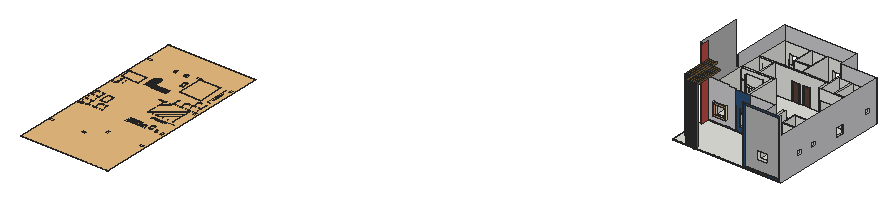
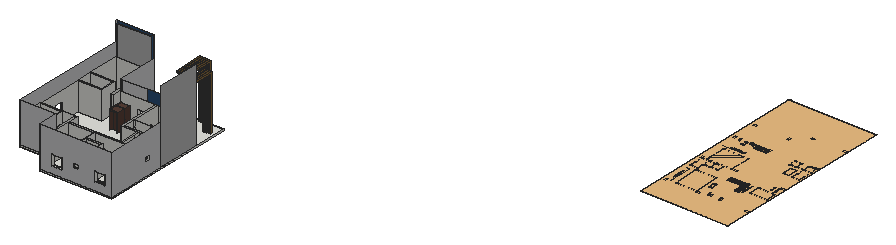
# SketchUp Ruby script. Lengths in inches.
U = 1.inch
M = Sketchup.active_model
def pt(a) = Geom::Point3d.new(a.map { |v| v * U })
def face(e, loops, mat)
  f = e.add_face(loops[0].map { |a| pt(a) })
  loops[1..].each { |l| e.add_face(l.map { |a| pt(a) }).erase! }
  f.material = f.back_material = mat if mat
  f
end
# faces: each face lists its corners as indices into pts; further lists are holes
def faces(e, pts, list, mat = nil) = list.each { |f| face(e, (f[0].is_a?(Array) ? f : [f]).map { |l| l.map { |i| pts[i] } }, mat) }
# xy, xz, yz: faces in a plane at the given z, y or x. An outline is a flat list of corners, or four numbers for a rectangle; further outlines are holes
def ring(l) = l.size == 4 ? [[l[0], l[1]], [l[2], l[1]], [l[2], l[3]], [l[0], l[3]]] : l.each_slice(2).to_a
def flat(e, list, mat, &to3) = list.each { |f| face(e, (f[0].is_a?(Array) ? f : [f]).map { |l| ring(l).map { |u, v| to3.(u, v) } }, mat) }
def xy(e, z, list, mat = nil) = flat(e, list, mat) { |x, y| [x, y, z] }
def xz(e, y, list, mat = nil) = flat(e, list, mat) { |x, z| [x, y, z] }
def yz(e, x, list, mat = nil) = flat(e, list, mat) { |y, z| [x, y, z] }
def lines(e, pts, list) = list.each { |a, b| e.add_line(pt(pts[a]), pt(pts[b])) }
# prism: a flat outline (further loops are holes) pulled along v
def prism(e, loops, v, mat = nil)
  f = face(e, loops, mat); d = Geom::Vector3d.new(v.map { |x| x * U })
  f.pushpull(f.normal.samedirection?(d) ? d.length : -d.length)
end
def box(e, o, s, mat = nil) = prism(e, [[o, [o[0] + s[0], o[1], o[2]], [o[0] + s[0], o[1] + s[1], o[2]], [o[0], o[1] + s[1], o[2]]]], [0, 0, s[2]], mat)
def at(x, y, z, deg = 0) = Geom::Transformation.translation(pt([x, y, z])) * Geom::Transformation.rotation(ORIGIN, Z_AXIS, deg.degrees)
def axes(o, x, y, z) = Geom::Transformation.new([*x, 0, *y, 0, *z, 0, *pt(o).to_a, 1])
def part(name) = M.definitions.add(name)
# library, detail: a bought-in or finely detailed component or shape, given as its bounding box
def library(name, o, s) = part(name).tap { |d| box(d.entities, o, s) }
def detail(e, o, s) = box(e.add_group.entities, o, s)
def put(e, d, t, mat = nil) = e.add_instance(d, t).tap { |i| i.material = mat if mat }
def group(e, t, mat = nil) = e.add_group.tap { |g| g.transformation = t; g.material = mat if mat }.entities
root = M.entities
M.materials.add("1dt57im4").color = [86, 62, 54]
M.materials.add("Heather_PantShadow").color = [42, 79, 119]
M.materials.add("Heather_Skin").color = [229, 155, 121]
M.materials.add("K359").color = [135, 104, 58]
M.materials.add("Material~76").color = [176, 176, 176]
M.materials.add("Panel-Opening1").color = [194, 151, 109]
M.materials.add("[Color_D05]").color = [255, 242, 204]
M.materials.add("[Metal Rusted]").color = [184, 75, 66]
M.materials.add("[Polished Concrete New]").color = [200, 200, 203]
c1 = part("345tyh")
p = [[-7.5,4.5,0],[7.5,4.5,0],[7.5,-4.5,0],[-7.5,-4.5,0]]
lines(c1.entities,p,[[0,1],[1,2],[2,3],[3,0]])
c2 = part("wertghj")
p = [[-196.8,-126,0],[-196.8,-117,0],[-178.8,-117,0],[-178.8,-126,0],[32.8,-126,0],[23.8,-126,0],
  [23.8,-108,0],[32.8,-108,0],[-196.8,70.5,0],[-196.8,79.5,0],[-178.8,79.5,0],[-178.8,70.5,0],
  [-196.8,282,0],[-196.8,291,0],[-178.8,291,0],[-178.8,282,0],[31.8,282,0],[31.8,291,0],
  [49.8,291,0],[49.8,282,0],[23.8,70.5,0],[23.8,79.5,0],[41.8,79.5,0],[41.8,70.5,0]]
lines(c2.entities,p,[[0,1],[1,2],[2,3],[3,0],[4,5],[5,6],[6,7],[7,4],[8,9],[9,10],[10,11],[11,8],
  [12,13],[13,14],[14,15],[15,12],[16,17],[17,18],[18,19],[19,16],[20,21],[21,22],[22,23],[23,20]])
put(c2.entities,c1,at(-189.3,-286.5,0))
put(c2.entities,c1,at(-39.2,-286.5,0))
put(c2.entities,c1,at(189.3,-234.5,0))
put(c2.entities,c1,at(192.3,-118.5,0,-90))
put(c2.entities,c1,at(192.3,72,0,90))
put(c2.entities,c1,at(192.3,283.5,0,90))
put(c2.entities,c1,at(28.3,-231.5,0,-90))
c3 = library("QWER",[-205.05,-433.25,0],[410.1,866.5,0.01])
c4 = library("DSKJFR",[-425,-425,0],[850,850,0.01])
c5 = library("DFKJR",[-425,-425,0],[850,850,0.01])
c6 = library("2W3ERTY",[-59.64,-49.54,0],[119.28,99.08,0.01])
c7 = library("A$C6BA60DA3",[-259.19,-49.25,0],[518.38,98.5,0.01])
c8 = library("QWERTYU",[-39.01,-24.72,0],[78.02,49.44,0.01])
c9 = library("MUDDA1",[-12.79,-16.5,0],[25.58,33.01,0.01])
c10 = part("WERTYYYY")
p = [[-172.05,43.88,0],[-172.05,-2.3,0],[-109.67,-98.49,0],[-139.58,-98.49,0],[-139.58,-147.08,0],[-109.67,-147.08,0],
  [-111.91,-100.73,0],[-137.33,-100.73,0],[-137.33,-144.84,0],[-111.91,-144.84,0],[181.78,172.12,0],[181.78,111.05,0],
  [185.12,111.05,0],[185.12,172.12,0],[185.12,122.5,0],[188.46,122.5,0],[188.46,162.08,0],[185.12,162.08,0],
  [190.05,87.18,0],[175.05,87.18,0],[175.05,200.2,0],[-52.95,111.7,0],[-52.95,44.2,0],[-52.95,68.2,0],
  [17.55,68.2,0],[-64.15,111.7,0],[-64.15,44.2,0],[-64.95,111.7,0],[-64.95,44.2,0],[17.55,44.2,0],
  [16,54.45,0],[-52.95,54.45,0],[16,55.24,0],[-52.95,55.24,0],[90.55,-123.8,0],[190.05,-123.8,0],
  [156.05,-129.06,0],[94.98,-129.06,0],[94.98,-132.4,0],[156.05,-132.4,0],[106.43,-132.4,0],[106.43,-135.75,0],
  [146.01,-135.75,0],[146.01,-132.4,0],[90.55,-138.8,0],[-88.14,106.88,0],[-88.14,45.82,0],[-84.79,45.82,0],
  [-84.79,106.88,0],[-84.79,57.27,0],[-81.45,57.27,0],[-81.45,96.84,0],[-84.79,96.84,0],[89,-191.27,0],
  [30.55,-191.27,0],[89,-190.47,0],[30.55,-190.47,0]]
lines(c10.entities,p,[[0,1],[2,3],[3,4],[4,5],[5,2],[6,7],[7,8],[8,9],[9,6],[10,11],[11,12],[12,13],
  [14,15],[15,16],[16,17],[17,14],[18,19],[19,20],[21,22],[23,24],[25,26],[27,28],[24,29],[30,31],
  [32,33],[34,35],[36,37],[37,38],[38,39],[40,41],[41,42],[42,43],[43,40],[34,44],[10,13],[45,46],
  [46,47],[47,48],[49,50],[50,51],[51,52],[52,49],[45,48],[36,39],[53,54],[55,56]])
put(c10.entities,c4,axes([-139.43,-181.93,0],[0.0397,0,0],[0,-0.0397,0],[0,0,0.0397]))
put(c10.entities,c5,axes([-173.18,-181.93,0],[0,0.0397,0],[-0.0397,0,0],[0,0,0.0397]))
put(c10.entities,c4,axes([-105.68,-181.93,0],[0.0397,0,0],[0,-0.0397,0],[0,0,0.0397]))
put(c10.entities,c4,axes([-173.18,-148.18,0],[0,-0.0397,0],[-0.0397,0,0],[0,0,0.0397]))
put(c10.entities,c4,axes([-173.18,-114.4375,0],[0,-0.0397,0],[-0.0397,0,0],[0,0,0.0397]))
put(c10.entities,c6,at(101.59,140.56,0,90))
put(c10.entities,c4,axes([139.43,14.57,0],[-0.0397,0,0],[0,-0.0397,0],[0,0,0.0397]))
put(c10.entities,c5,axes([173.18,14.57,0],[0,0.0397,0],[0.0397,0,0],[0,0,0.0397]))
put(c10.entities,c4,axes([105.68,14.57,0],[-0.0397,0,0],[0,-0.0397,0],[0,0,0.0397]))
put(c10.entities,c4,axes([173.18,48.32,0],[0,-0.0397,0],[0.0397,0,0],[0,0,0.0397]))
put(c10.entities,c7,axes([-64.49,63.07,0],[0.03573,0,0],[0,-0.03573,0],[0,0,0.03573]))
put(c10.entities,c7,axes([-64.49,59.6,0],[0.03573,0,0],[0,-0.03573,0],[0,0,0.03573]))
put(c10.entities,c7,axes([-64.49,56.14,0],[0.03573,0,0],[0,-0.03573,0],[0,0,0.03573]))
put(c10.entities,c7,axes([-64.49,52.35,0],[0.03573,0,0],[0,-0.03573,0],[0,0,0.03573]))
put(c10.entities,c7,axes([-64.49,96.62,0],[0.03573,0,0],[0,-0.03573,0],[0,0,0.03573]))
put(c10.entities,c7,axes([-64.49,93.16,0],[0.03573,0,0],[0,-0.03573,0],[0,0,0.03573]))
put(c10.entities,c7,axes([-64.49,89.69,0],[0.03573,0,0],[0,-0.03573,0],[0,0,0.03573]))
put(c10.entities,c7,axes([-64.49,86.22,0],[0.03573,0,0],[0,-0.03573,0],[0,0,0.03573]))
put(c10.entities,c7,axes([-64.49,82.76,0],[0.03573,0,0],[0,-0.03573,0],[0,0,0.03573]))
put(c10.entities,c7,axes([-64.49,79.29,0],[0.03573,0,0],[0,-0.03573,0],[0,0,0.03573]))
put(c10.entities,c7,axes([-64.49,75.83,0],[0.03573,0,0],[0,-0.03573,0],[0,0,0.03573]))
put(c10.entities,c7,axes([-64.49,66.53,0],[0.03573,0,0],[0,-0.03573,0],[0,0,0.03573]))
put(c10.entities,c7,axes([-64.49,73.02,0],[0.03573,0,0],[0,-0.03573,0],[0,0,0.03573]))
put(c10.entities,c7,axes([-64.49,69.56,0],[0.03573,0,0],[0,-0.03573,0],[0,0,0.03573]))
put(c10.entities,c7,axes([-64.49,102.59,0],[0.03573,0,0],[0,-0.03573,0],[0,0,0.03573]))
put(c10.entities,c7,axes([-64.49,99.21,0],[0.03573,0,0],[0,-0.03573,0],[0,0,0.03573]))
put(c10.entities,c7,axes([-64.49,49.1,0],[0.03573,0,0],[0,-0.03573,0],[0,0,0.03573]))
put(c10.entities,c7,axes([-25.13,54.78,0],[0,-0.03573,0],[-0.03573,0,0],[0,0,0.03573]))
put(c10.entities,c7,axes([-28.6,54.78,0],[0,-0.03573,0],[-0.03573,0,0],[0,0,0.03573]))
put(c10.entities,c7,axes([-32.0625,54.78,0],[0,-0.03573,0],[-0.03573,0,0],[0,0,0.03573]))
put(c10.entities,c7,axes([-35.85,54.78,0],[0,-0.03573,0],[-0.03573,0,0],[0,0,0.03573]))
put(c10.entities,c7,axes([8.42,54.78,0],[0,-0.03573,0],[-0.03573,0,0],[0,0,0.03573]))
put(c10.entities,c7,axes([4.96,54.78,0],[0,-0.03573,0],[-0.03573,0,0],[0,0,0.03573]))
put(c10.entities,c7,axes([1.49,54.78,0],[0,-0.03573,0],[-0.03573,0,0],[0,0,0.03573]))
put(c10.entities,c7,axes([-1.97,54.78,0],[0,-0.03573,0],[-0.03573,0,0],[0,0,0.03573]))
put(c10.entities,c7,axes([-5.4375,54.78,0],[0,-0.03573,0],[-0.03573,0,0],[0,0,0.03573]))
put(c10.entities,c7,axes([-8.9,54.78,0],[0,-0.03573,0],[-0.03573,0,0],[0,0,0.03573]))
put(c10.entities,c7,axes([-12.37,54.78,0],[0,-0.03573,0],[-0.03573,0,0],[0,0,0.03573]))
put(c10.entities,c7,axes([-21.67,54.78,0],[0,-0.03573,0],[-0.03573,0,0],[0,0,0.03573]))
put(c10.entities,c7,axes([-15.17,54.78,0],[0,-0.03573,0],[-0.03573,0,0],[0,0,0.03573]))
put(c10.entities,c7,axes([-18.64,54.78,0],[0,-0.03573,0],[-0.03573,0,0],[0,0,0.03573]))
put(c10.entities,c7,axes([14.39,54.78,0],[0,-0.03573,0],[-0.03573,0,0],[0,0,0.03573]))
put(c10.entities,c7,axes([11.01,54.78,0],[0,-0.03573,0],[-0.03573,0,0],[0,0,0.03573]))
put(c10.entities,c7,axes([-39.1,54.78,0],[0,-0.03573,0],[-0.03573,0,0],[0,0,0.03573]))
put(c10.entities,c7,axes([-42.1875,54.78,0],[0,-0.03573,0],[-0.03573,0,0],[0,0,0.03573]))
put(c10.entities,c7,axes([-45.4375,54.78,0],[0,-0.03573,0],[-0.03573,0,0],[0,0,0.03573]))
put(c10.entities,c7,axes([-48.46,54.78,0],[0,-0.03573,0],[-0.03573,0,0],[0,0,0.03573]))
put(c10.entities,c7,axes([-50.9,54.78,0],[0,-0.03573,0],[-0.03573,0,0],[0,0,0.03573]))
put(c10.entities,c7,axes([-64.49,109.94,0],[0.03573,0,0],[0,-0.03573,0],[0,0,0.03573]))
put(c10.entities,c7,axes([-64.49,106.56,0],[0.03573,0,0],[0,-0.03573,0],[0,0,0.03573]))
put(c10.entities,c6,at(110.65,-56.34,0))
put(c10.entities,c8,at(-151.04,67.61,0))
put(c10.entities,c9,axes([-168.97,17.91,0],[0,-0.75735,0],[-0.75735,0,0],[0,0,0.75735]))
put(c10.entities,c7,axes([47.87,-190.9375,0],[0,-0.03573,0],[-0.03573,0,0],[0,0,0.03573]))
put(c10.entities,c7,axes([44.4,-190.9375,0],[0,-0.03573,0],[-0.03573,0,0],[0,0,0.03573]))
put(c10.entities,c7,axes([40.9375,-190.9375,0],[0,-0.03573,0],[-0.03573,0,0],[0,0,0.03573]))
put(c10.entities,c7,axes([37.15,-190.9375,0],[0,-0.03573,0],[-0.03573,0,0],[0,0,0.03573]))
put(c10.entities,c7,axes([81.42,-190.94,0],[0,-0.03573,0],[-0.03573,0,0],[0,0,0.03573]))
put(c10.entities,c7,axes([77.96,-190.94,0],[0,-0.03573,0],[-0.03573,0,0],[0,0,0.03573]))
put(c10.entities,c7,axes([74.49,-190.94,0],[0,-0.03573,0],[-0.03573,0,0],[0,0,0.03573]))
put(c10.entities,c7,axes([71.03,-190.94,0],[0,-0.03573,0],[-0.03573,0,0],[0,0,0.03573]))
put(c10.entities,c7,axes([67.5625,-190.94,0],[0,-0.03573,0],[-0.03573,0,0],[0,0,0.03573]))
put(c10.entities,c7,axes([64.1,-190.94,0],[0,-0.03573,0],[-0.03573,0,0],[0,0,0.03573]))
put(c10.entities,c7,axes([60.63,-190.94,0],[0,-0.03573,0],[-0.03573,0,0],[0,0,0.03573]))
put(c10.entities,c7,axes([51.33,-190.9375,0],[0,-0.03573,0],[-0.03573,0,0],[0,0,0.03573]))
put(c10.entities,c7,axes([57.83,-190.9375,0],[0,-0.03573,0],[-0.03573,0,0],[0,0,0.03573]))
put(c10.entities,c7,axes([54.36,-190.9375,0],[0,-0.03573,0],[-0.03573,0,0],[0,0,0.03573]))
put(c10.entities,c7,axes([87.39,-190.94,0],[0,-0.03573,0],[-0.03573,0,0],[0,0,0.03573]))
put(c10.entities,c7,axes([84.01,-190.94,0],[0,-0.03573,0],[-0.03573,0,0],[0,0,0.03573]))
put(c10.entities,c7,axes([33.9,-190.9375,0],[0,-0.03573,0],[-0.03573,0,0],[0,0,0.03573]))
c11 = library("basin11",[-225,-150,0],[450,300,0.01])
c12 = library("closet2",[-315,-170,0],[630,340,0.01])
c13 = library("Shower",[-145.23,-92.17,0],[290.46,184.34,0.01])
c14 = part("A$C31335114")
p = [[8.96,-126.88,0],[8.96,-85.95,0],[-26.04,-126.88,0],[-26.04,-85.95,0],[-68.45,-139.23,0],[-106.23,-139.23,0],
  [-106.23,-127.73,0],[-68.45,-127.73,0],[-31.54,-127.73,0],[-87.34,-115.75,0],[-26.04,-115.67,0],[-87.34,-127.73,0],
  [-54.82,-145.23,0],[-119.82,-145.23,0],[-119.82,-139.23,0],[-54.82,-139.23,0]]
lines(c14.entities,p,[[0,1],[2,3],[4,5],[5,6],[6,7],[7,4],[7,8],[9,10],[11,9],[12,13],[13,14],[14,15],
  [15,12]])
put(c14.entities,c13,axes([27.65,0,0],[0,1,0],[1,0,0],[0,0,1]))
c15 = part("WERTGTTY")
put(c15.entities,c11,axes([-60.92,193.38,0],[0.03936,0,0],[0,0.03936,0],[0,0,0.03936]))
put(c15.entities,c12,axes([-26.2,135.1,0],[0,-0.03936,0],[0.03936,0,0],[0,0,0.03936]))
put(c15.entities,c11,axes([52.43,-195.4,0],[0.03936,0,0],[0,-0.03936,0],[0,0,0.03936]))
put(c15.entities,c12,axes([80.29,-184.4,0],[0,-0.03936,0],[-0.03936,0,0],[0,0,0.03936]))
put(c15.entities,c14,axes([111.86,-195.53,0],[-0.0397,0,0],[0,0.0397,0],[0,0,0.0397]))
put(c15.entities,c14,axes([-111.86,195.53,0],[0.0397,0,0],[0,-0.0397,0],[0,0,0.0397]))
c16 = part("First Floor Plan.dwg")
put(c16.entities,c2,at(201.3,455.5,0))
put(c16.entities,c3,at(205.05,433.25,0))
put(c16.entities,c10,at(199.05,537.3,0))
put(c16.entities,c15,at(254.8,535.3,0))
c17 = part("Door panel")
xy(c17.entities,0,[[0,0,0,1.5,42,1.5,42,0,38.18,0,38.18,0.5,3.82,0.5,3.82,0]],"1dt57im4")
xy(c17.entities,74.18,[[3.82,0,38.18,0.5]],"1dt57im4")
xy(c17.entities,78,[[0,0,42,1.5]],"1dt57im4")
xz(c17.entities,0,[[0,0,3.82,0,3.82,74.18,38.18,74.18,38.18,0,42,0,42,78,0,78]],"1dt57im4")
xz(c17.entities,0.5,[[3.82,0,38.18,74.18]],"1dt57im4")
xz(c17.entities,1.5,[[0,0,42,78]])
yz(c17.entities,0,[[0,0,1.5,78]],"1dt57im4")
yz(c17.entities,3.82,[[0,0,0.5,74.18]],"1dt57im4")
yz(c17.entities,38.18,[[0,0,0.5,74.18]],"1dt57im4")
yz(c17.entities,42,[[0,0,1.5,78]],"1dt57im4")
c18 = part("Untitled (2)")
g1 = group(c18.entities,at(0,0,0))
put(g1,c17,axes([0,3,0],[1,0,0],[0,-1,0],[0,0,1]))
put(g1,c17,at(0,0,0))
xy(root,-10.62,[[42.76,58.375,48.94,63.6]],"K359")
xy(root,-9.93,[[31.92,58.375,38.11,63.6]],"K359")
xy(root,-9.43,[[21.24,58.375,27.43,63.6]],"K359")
xy(root,-6.12,[[52.37,58.375,58.56,63.6]],"K359")
xy(root,0,[[[3.9,8.875,3.9,661.375,342.9,661.375,342.9,565.375,510.9,565.375,510.9,8.875],[98.86,9.52,105.05,14.74],[21.24,58.375,27.43,63.6],[31.92,58.375,38.11,63.6],[42.76,58.375,48.94,63.6]],[98.86,9.52,105.05,14.74],[21.24,58.375,27.43,63.6],[31.92,58.375,38.11,63.6],[42.76,58.375,48.94,63.6]],"K359")
xy(root,0.63,[[52.37,58.375,58.56,63.6]],"K359")
xy(root,0.6875,[[88.02,9.52,94.21,14.74]],"K359")
xy(root,1.1875,[[77.35,9.52,83.53,14.74]],"K359")
xy(root,1.3125,[[65.39,9.52,73.21,14.74]],"K359")
xy(root,1.8,[[9.01,164.8125,15.77,196.375]],"[Metal Rusted]")
xy(root,4.5,[[108.47,9.52,114.66,14.74]],"K359")
xy(root,6,[[3.9,8.875,336.9,8.875,336.9,196.375,9.01,196.375,9.01,381.48,3.9,381.48],[336.9,8.875,336.9,196.375,342.9,196.375,342.9,241.375,345.9,241.375,345.9,17.875,404.62,17.875,404.62,8.875],[404.62,8.875,440.62,17.875],[440.62,8.875,440.62,17.875,501.9,17.875,501.9,131.875,510.9,131.875,510.9,8.875],[501.9,131.875,501.9,161.875,425.4,161.875,425.4,167.875,501.9,167.875,501.9,182.875,510.9,182.875,510.9,131.875],
  [501.9,182.875,510.9,212.875],[9.01,196.375,9.01,381.48,3.9,381.48,3.9,406.375,17.9,406.375,17.9,397.41,12.9,397.41,12.9,205.375,51.9,205.375,51.9,196.375],[51.9,196.375,99.9,205.375],[99.9,196.375,99.9,205.375,156.9,205.375,156.9,397.375,150.9,397.375,150.9,406.375,165.9,406.375,165.9,196.375],[165.9,196.375,177.5,205.375],
  [177.5,196.375,249.5,205.375],[249.5,196.375,287.9,205.375],[327.9,196.375,327.9,205.375,333.9,205.375,333.9,241.375,342.9,241.375,342.9,196.375],[501.9,327.95,510.9,375.95],[501.9,375.95,501.9,451.375,399.9,451.375,399.9,464.375,405.9,464.375,405.9,460.375,501.9,460.375,501.9,496.375,510.9,496.375,510.9,375.95],
  [47.9,397.375,110.9,406.375],[3.9,406.375,12.9,439.375],[84.9,406.375,84.9,499.375,12.9,499.375,12.9,469.375,3.9,469.375,3.9,661.375,12.9,661.375,12.9,508.375,167.9,508.375,167.9,499.375,90.9,499.375,90.9,406.375],[3.9,439.375,12.9,469.375],[333.9,451.375,333.9,499.375,253.9,499.375,253.9,508.375,342.9,508.375,342.9,451.375],
  [399.9,494.375,399.9,556.375,342.9,556.375,342.9,565.375,510.9,565.375,510.9,526.375,501.9,526.375,501.9,556.375,405.9,556.375,405.9,494.375],[501.9,496.375,510.9,526.375],[203.9,499.375,217.9,508.375],[207.9,508.375,207.9,556.375,203.9,556.375,203.9,562.375,207.9,562.375,207.9,652.375,188.71,652.375,188.71,661.375,237.9,661.375,237.9,652.375,213.9,652.375,213.9,508.375],[333.9,508.375,333.9,652.375,285.9,652.375,285.9,661.375,342.9,661.375,342.9,508.375],
  [132.9,556.375,132.9,652.375,84.9,652.375,84.9,661.375,158.71,661.375,158.71,652.375,138.9,652.375,138.9,562.375,173.9,562.375,173.9,556.375],[12.9,652.375,36.9,661.375],[36.9,652.375,84.9,661.375],[158.71,652.375,188.71,661.375],[237.9,652.375,285.9,661.375]])
xy(root,6,[[336.9,0,404.62,8.875],[404.62,0,440.62,8.875],[440.62,0,510.9,8.875]],"Heather_PantShadow")
xy(root,11.38,[[150.06,191.8125,165.9,196.375]],"[Metal Rusted]")
xy(root,12,[[342.9,0,504.9,8.875]],"Heather_PantShadow")
xy(root,16.62,[[60.01,357.52,69.01,390.52],[60.01,390.52,69.01,420.52],[69.01,603.52,93.01,612.52],[93.01,603.52,141.01,612.52]])
xy(root,36,[[45.9,190.375,105.9,196.375]],"[Color_D05]")
xy(root,36.1875,[[171.5,190.375,216.36,196.375],[216.36,190.375,255.5,196.375]],"[Color_D05]")
xy(root,42,[[51.9375,190.375,99.9,190.375,99.9,205.375,51.9,205.375,51.9,196.375,51.9375,196.375],[177.5,190.375,249.5,205.375],[501.9,327.95,510.9,375.95],[36.9,652.375,84.9,661.375],[237.9,652.375,285.9,661.375]])
xy(root,42,[[51.9,190.375,51.9375,196.375]],"Heather_Skin")
xy(root,100.62,[[74.01,348.52,104.01,357.52]])
xz(root,0,[[[336.9,6,510.9,280.6875],[342.9,12,504.9,274.0625]]],"Heather_PantShadow")
xz(root,8.875,[[3.9,0,336.9,6],[336.9,0,510.9,6]])
xz(root,8.875,[[[342.9,12,504.9,274.0625],[398.62,54,446.62,96]]],"Material~76")
xz(root,9.52,[[98.86,0,105.05,273.5],[88.02,0.6875,94.21,273.5],[77.35,1.1875,83.53,273.5],[65.39,1.3125,73.21,273.5],[108.47,4.5,114.66,273.5]],"K359")
xz(root,14.74,[[98.86,0,105.05,267.3125],[88.02,0.6875,94.21,267.3125],[77.35,1.1875,83.53,267.3125],[65.39,1.3125,73.21,267.3125],[108.47,4.5,114.66,267.3125]],"K359")
xz(root,17.875,[[[345.9,6,501.9,138],[404.62,60,440.62,90]]])
xz(root,58.375,[[42.76,-10.62,48.94,0],[31.92,-9.93,38.11,0],[21.24,-9.43,27.43,0],[52.37,-6.12,58.56,0.63],[21.24,0,27.43,262.88],
  [31.92,0,38.11,262.88],[42.76,0,48.94,262.88],[52.37,0.63,58.56,262.88]],"K359")
xz(root,63.6,[[42.76,-10.62,48.94,0],[31.92,-9.93,38.11,0],[21.24,-9.43,27.43,0],[52.37,-6.12,58.56,0.63],[21.24,0,27.43,256.7],
  [31.92,0,38.11,256.7],[42.76,0,48.94,256.7],[52.37,0.63,58.56,256.7]],"K359")
xz(root,161.875,[[389.4,6,395.4,6,395.4,90,425.4,90,425.4,6,501.9,6,501.9,138,389.4,138]])
xz(root,164.8125,[[9.01,1.8,15.77,343.875]],"[Metal Rusted]")
xz(root,167.875,[[425.4,6,425.4,90,395.4,90,395.4,138,501.9,138,501.9,6]])
xz(root,190.375,[[[45.9,36,105.9,96.08],[51.9,42,99.9,90]],[[171.5,36.1875,255.5,96.18],[177.5,42,249.5,90]]],"Panel-Opening1")
xz(root,191.8125,[[150.06,11.38,165.9,11.38,216.47,11.6,216.36,36.1875,171.5,36,171.5,36.1875,171.25,96.2,165.55,96.18,165.5,108.3125,165.55,108.3125,165.55,108.37,171.5,108.37,171.5,96.18,216.0625,96.18,216.0625,181.375,150.19,181.375,150.19,116.53,150.06,116.53]],"Heather_PantShadow")
xz(root,196.375,[[51.9,42,51.9375,89.91]])
xz(root,196.375,[[9.29,6,15.77,11.38],[15.77,6,287.9,6,287.9,90,327.9,90,327.9,6,336.9,6,336.9,181.375,331.52,181.375,331.52,95.38,282.52,95.38,282.52,11.38,15.77,11.38]],"Heather_PantShadow")
xz(root,196.375,[[9.01,1.8,9.29,6],[9.29,1.8,15.77,6]],"[Metal Rusted]")
xz(root,196.375,[[9.29,11.38,15.77,189.3],[[15.77,11.38,150.06,11.38,150.06,181.78,114.62,181.78,114.62,189.3,15.77,189.3],[45.9,36,105.9,96.08]],[165.9,11.38,282.52,11.38,282.52,95.38,331.52,95.38,331.52,181.375,216.0625,181.375,216.0625,96.18,255.5,96.18,255.5,36.1875,171.5,36.1875,171.5,108.37,165.55,108.37,165.55,96.18,171.25,96.2,171.5,36.1875,171.5,36,216.36,36.1875,216.47,11.6]],"[Polished Concrete New]")
xz(root,205.375,[[[12.9,6,156.9,138],[51.9,42,99.9,90]],[[165.9,6,165.9,138,333.9,138,333.9,6,327.9,6,327.9,90,287.9,90,287.9,6],[177.5,42,249.5,90]]])
xz(root,235.375,[[395.4,6,501.9,138]])
xz(root,241.375,[[333.9,6,345.9,138],[389.4,6,501.9,138]])
xz(root,327.95,[[501.9,42,510.9,90]])
xz(root,348.55,[[69.01,16.62,74.01,148.62]])
xz(root,357.52,[[69.01,16.62,69.01,148.62,141.01,148.62,141.01,16.62,104.01,16.62,104.01,100.62,74.01,100.62,74.01,16.62],[141.01,16.62,147.01,148.62]])
xz(root,375.95,[[501.9,42,510.9,90]])
xz(root,381.48,[[3.9,6,9.01,194.6875]],"Heather_PantShadow")
xz(root,397.375,[[47.9,6,110.9,6,110.9,90,150.9,90,150.9,6,156.9,6,156.9,138,17.9,138,17.9,90,47.9,90]])
xz(root,397.41,[[12.9,6,17.9,138]])
xz(root,406.375,[[12.9,6,12.9,138,84.9,138,84.9,6,47.9,6,47.9,90,17.9,90,17.9,6],[84.9,6,90.9,138],[90.9,6,90.9,138,165.9,138,165.9,6,150.9,6,150.9,90,110.9,90,110.9,6]])
xz(root,451.375,[[333.9,6,342.9,6,342.9,90,399.9,90,399.9,6,501.9,6,501.9,138,333.9,138]])
xz(root,460.375,[[405.9,6,501.9,138]])
xz(root,464.375,[[399.9,6,405.9,42],[399.9,42,405.9,90]])
xz(root,494.375,[[399.9,6,405.9,90]])
xz(root,499.375,[[12.9,6,84.9,138],[90.9,6,167.9,6,167.9,90,203.9,90,203.9,6,217.9,6,217.9,90,253.9,90,253.9,6,333.9,6,333.9,138,90.9,138]])
xz(root,508.375,[[12.9,6,12.9,138,207.9,138,207.9,6,203.9,6,203.9,90,167.9,90,167.9,6],[213.9,6,213.9,138,333.9,138,333.9,6,253.9,6,253.9,90,217.9,90,217.9,6]])
xz(root,556.375,[[132.9,6,173.9,6,173.9,90,203.9,90,203.9,6,207.9,6,207.9,138,132.9,138],[342.9,6,399.9,138],[405.9,6,501.9,138]])
xz(root,562.375,[[138.9,6,138.9,138,207.9,138,207.9,6,203.9,6,203.9,90,173.9,90,173.9,6]])
xz(root,565.375,[[342.9,0,510.9,6]])
xz(root,565.375,[[342.9,6,510.9,194.6875]],"[Polished Concrete New]")
xz(root,652.375,[[[12.9,6,132.9,138],[36.9,42,84.9,90]],[[138.9,6,207.9,138],[158.71,66,188.71,90]],[[213.9,6,333.9,138],[237.9,42,285.9,90]]])
xz(root,661.375,[[3.9,0,342.9,6]])
xz(root,661.375,[[[3.9,6,342.9,194.6875],[36.9,42,84.9,90],[237.9,42,285.9,90],[158.71,66,188.71,90]]],"[Polished Concrete New]")
yz(root,3.9,[[8.875,0,661.375,6]])
yz(root,3.9,[[[381.48,6,661.375,194.6875],[439.375,66,469.375,90]]],"[Polished Concrete New]")
yz(root,9.01,[[164.8125,1.8,196.375,1.8,196.375,6,381.48,6,381.48,146.6875,372.48,146.6875,372.48,343.875,164.8125,343.875]],"Material~76")
yz(root,12.9,[[205.375,6,397.375,138],[397.375,6,397.41,138],[[406.375,6,499.375,138],[439.375,66,469.375,90]],[508.375,6,652.375,138]])
yz(root,15.77,[[164.8125,1.8,196.375,335.23]],"[Metal Rusted]")
yz(root,17.9,[[397.33,6,397.41,6,397.41,90,397.375,90],[397.41,6,406.375,90]])
yz(root,21.24,[[58.375,-9.43,63.6,0],[58.375,0,58.375,262.88,196.375,262.88,196.375,256.7,63.6,256.7,63.6,0]],"K359")
yz(root,27.43,[[58.375,-9.43,63.6,0],[58.375,0,63.6,0,63.6,256.7,196.375,256.7,196.375,262.88,58.375,262.88]],"K359")
yz(root,31.92,[[58.375,-9.93,63.6,0],[58.375,0,58.375,262.88,196.375,262.88,196.375,256.7,63.6,256.7,63.6,0]],"K359")
yz(root,36.9,[[652.375,42,661.375,90]])
yz(root,38.11,[[58.375,-9.93,63.6,0],[58.375,0,63.6,0,63.6,256.7,196.375,256.7,196.375,262.88,58.375,262.88]],"K359")
yz(root,42.76,[[58.375,-10.62,63.6,0],[58.375,0,58.375,262.88,196.375,262.88,196.375,256.7,63.6,256.7,63.6,0]],"K359")
yz(root,45.9,[[190.375,36,196.375,96.08]],"[Color_D05]")
yz(root,47.9,[[397.33,6,397.375,42],[397.375,6,406.375,42],[397.375,42,406.375,90]])
yz(root,48.94,[[58.375,-10.62,63.6,0],[58.375,0,63.6,0,63.6,256.7,196.375,256.7,196.375,262.88,58.375,262.88]],"K359")
yz(root,51.9,[[196.375,42,205.375,90]])
yz(root,51.9,[[190.375,42,196.375,89.91]],"Heather_Skin")
yz(root,52.37,[[58.375,-6.12,63.6,0.63],[58.375,0.63,58.375,262.88,196.375,262.88,196.375,256.7,63.6,256.7,63.6,0.63]],"K359")
yz(root,58.56,[[58.375,-6.12,63.6,0.63],[58.375,0.63,63.6,0.63,63.6,256.7,196.375,256.7,196.375,262.88,58.375,262.88]],"K359")
yz(root,65.39,[[9.52,1.3125,9.52,273.5,147.52,273.5,147.52,267.3125,14.74,267.3125,14.74,1.3125]],"K359")
yz(root,69.01,[[348.52,16.62,348.55,148.62]])
yz(root,73.21,[[9.52,1.3125,14.74,1.3125,14.74,267.3125,147.52,267.3125,147.52,273.5,9.52,273.5]],"K359")
yz(root,74.01,[[348.47,16.62,348.55,16.62,348.55,100.62,348.52,100.62],[348.55,16.62,357.52,100.62],[348.52,100.62,348.55,148.62]])
yz(root,77.35,[[9.52,1.1875,9.52,273.5,147.52,273.5,147.52,267.3125,14.74,267.3125,14.74,1.1875]],"K359")
yz(root,83.53,[[9.52,1.1875,14.74,1.1875,14.74,267.3125,147.52,267.3125,147.52,273.5,9.52,273.5]],"K359")
yz(root,84.9,[[406.375,6,499.375,138],[652.375,42,661.375,90]])
yz(root,88.02,[[9.52,0.6875,9.52,273.5,147.52,273.5,147.52,267.3125,14.74,267.3125,14.74,0.6875]],"K359")
yz(root,90.9,[[406.375,6,499.375,138]])
yz(root,94.21,[[9.52,0.6875,14.74,0.6875,14.74,267.3125,147.52,267.3125,147.52,273.5,9.52,273.5]],"K359")
yz(root,98.86,[[9.52,0,9.52,273.5,147.52,273.5,147.52,267.3125,14.74,267.3125,14.74,0]],"K359")
yz(root,99.9,[[190.375,42,190.375,89.91,196.375,89.91,196.375,90,205.375,90,205.375,42]])
yz(root,104.01,[[348.47,16.62,348.52,52.62],[348.52,16.62,357.52,52.62],[348.52,52.62,357.52,100.62]])
yz(root,105.05,[[9.52,0,14.74,0,14.74,267.3125,147.52,267.3125,147.52,273.5,9.52,273.5]],"K359")
yz(root,105.9,[[190.375,36,196.375,96.08]],"[Color_D05]")
yz(root,108.47,[[9.52,4.5,9.52,273.5,147.52,273.5,147.52,267.3125,14.74,267.3125,14.74,4.5]],"K359")
yz(root,110.9,[[397.375,6,406.375,90]])
yz(root,114.66,[[9.52,4.5,14.74,4.5,14.74,267.3125,147.52,267.3125,147.52,273.5,9.52,273.5]],"K359")
yz(root,132.9,[[556.375,6,652.375,138]])
yz(root,138.9,[[562.375,6,652.375,138]])
yz(root,150.06,[[191.8125,11.38,196.375,116.53]],"[Metal Rusted]")
yz(root,150.9,[[397.375,6,406.375,90]])
yz(root,156.9,[[205.375,6,397.375,138]])
yz(root,165.9,[[205.375,6,406.375,138]])
yz(root,167.9,[[499.375,6,508.375,90]])
yz(root,171.5,[[190.375,36.1875,190.375,96.18,191.8125,96.18,191.8125,108.37,196.375,108.37,196.375,36.1875]],"[Color_D05]")
yz(root,171.5,[[191.8125,36,196.375,36.1875]],"[Metal Rusted]")
yz(root,173.9,[[556.375,6,562.375,90]])
yz(root,177.5,[[190.375,42,205.375,90]])
yz(root,203.9,[[499.375,6,508.375,90],[556.375,6,562.375,90]])
yz(root,207.9,[[508.375,6,556.375,138],[562.375,6,652.375,138]])
yz(root,213.9,[[508.375,6,652.375,138]])
yz(root,217.9,[[499.375,6,508.375,90]])
yz(root,237.9,[[652.375,42,661.375,90]])
yz(root,249.5,[[190.375,42,205.375,90]])
yz(root,253.9,[[499.375,6,508.375,90]])
yz(root,255.5,[[190.375,36.1875,196.375,96.18]],"[Color_D05]")
yz(root,285.9,[[652.375,42,661.375,90]])
yz(root,287.9,[[196.375,6,205.375,90]])
yz(root,327.9,[[196.375,6,205.375,90]])
yz(root,333.9,[[205.375,6,241.375,138],[451.375,6,499.375,138],[508.375,6,652.375,138]])
yz(root,336.9,[[0,6,196.375,181.375]],"[Polished Concrete New]")
yz(root,342.9,[[565.375,0,661.375,6],[451.375,6,556.375,6,556.375,138,460.375,138,460.375,90,451.375,90]])
yz(root,342.9,[[0,12,8.875,274.0625]],"Heather_PantShadow")
yz(root,342.9,[[565.375,6,661.375,194.6875]],"[Polished Concrete New]")
yz(root,345.9,[[17.875,6,241.375,138]])
yz(root,389.4,[[161.875,6,241.375,138]])
yz(root,395.4,[[161.875,6,235.375,6,235.375,138,167.875,138,167.875,90,161.875,90]])
yz(root,399.9,[[451.375,6,451.375,90,460.375,90,460.375,138,556.375,138,556.375,6,494.375,6,494.375,90,464.375,90,464.375,6]])
yz(root,405.9,[[460.375,6,464.375,6,464.375,90,494.375,90,494.375,6,556.375,6,556.375,138,460.375,138]])
yz(root,425.4,[[161.875,6,167.875,90]])
yz(root,501.9,[[[17.875,6,161.875,138],[101.875,66,131.875,90]],[167.875,6,167.875,138,235.375,138,235.375,6,182.875,6,182.875,66,212.875,66,212.875,90,182.875,90,182.875,6],[[241.375,6,451.375,138],[327.95,42,375.95,90]],[[460.375,6,556.375,138],[496.375,66,526.375,90]]])
yz(root,504.9,[[0,12,8.875,274.0625]],"Heather_PantShadow")
yz(root,510.9,[[[8.875,0,565.375,0,565.375,194.6875,8.875,194.6875,8.875,280.6875,0,280.6875,0,6,8.875,6],[327.95,42,375.95,90],[101.875,66,131.875,90],[182.875,66,212.875,90],[496.375,66,526.375,90]]],"[Polished Concrete New]")
p = [[165.9,191.8125,11.38],[165.9,196.375,11.38],[216.47,196.375,11.6],[216.47,191.8125,11.6],[216.36,196.375,36.1875],[216.36,191.8125,36.1875],
  [171.5,196.375,36],[171.5,191.8125,36],[171.25,196.375,96.2],[171.25,191.8125,96.2],[171.5,191.8125,36.1875],[171.5,196.375,36.1875],
  [69.01,603.52,16.62],[69.01,459.52,16.62],[69.01,450.52,16.62],[69.01,450.52,148.62],[69.01,603.52,100.62],[69.01,420.52,16.62],
  [60.01,612.52,16.62],[60.01,420.52,16.62],[60.01,612.52,10.62],[69.01,612.52,16.62],[171.6,190.375,11.41],[255.5,190.375,11.41],
  [255.5,196.375,11.41]]
faces(root,p,[[0,1,2,3],[3,2,4,5],[6,7,5,4],[8,9,10,11]],"[Metal Rusted]")
lines(root,p,[[12,13],[14,15],[12,16],[17,14],[18,19],[20,18],[21,18],[22,23],[23,24]])
put(root,c16,at(-1876.15,-1457.92,0))
put(root,c18,axes([253.72,504.79,4.3],[-0.87429,0,0],[0,-1.02,0],[0,0,1.1118]))
put(root,c18,axes([167.18,504.44,6],[0.87429,0,0],[0,-1.02,0],[0,0,1.1118]))
g2 = group(root,at(0,6.17,6))
xy(g2,0,[[333,0,507,0,507,556.5,339,556.5,339,652.5,0,652.5,0,187.5,333,187.5]])
put(root,c18,axes([110.88,397.375,6],[0.95297,0,0],[0,0.27795,0],[0,0,1.10279]))
put(root,c18,axes([287.9,272.65,6],[0.95238,0,0],[0,-25.4252,0],[0,0,1.10395]))
